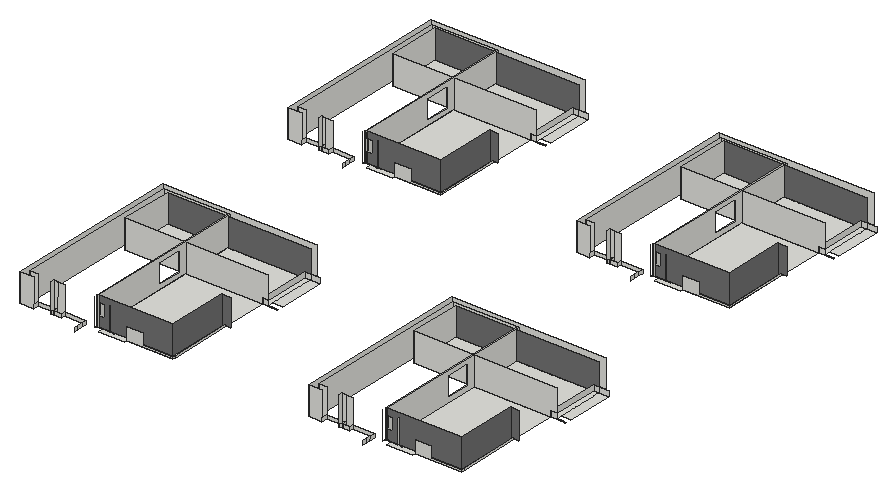
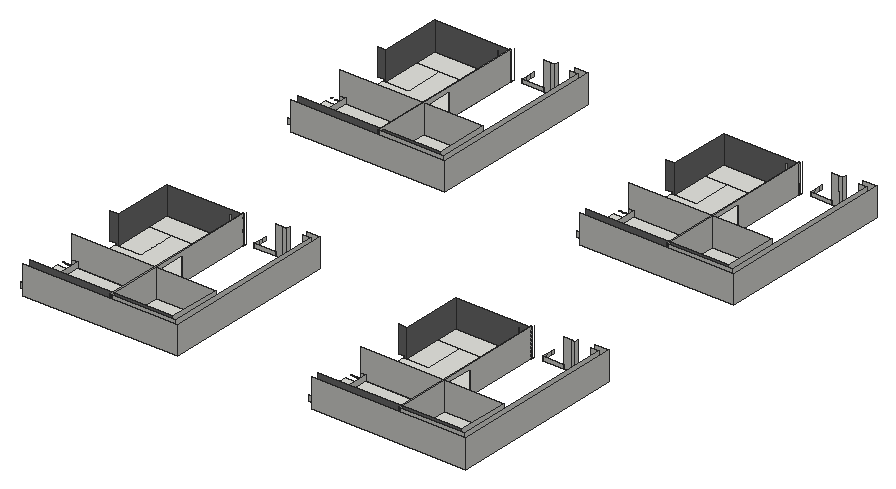
# SketchUp Ruby script. Lengths in inches.
U = 1.inch
M = Sketchup.active_model
def pt(a) = Geom::Point3d.new(a.map { |v| v * U })
def face(e, loops, mat)
  f = e.add_face(loops[0].map { |a| pt(a) })
  loops[1..].each { |l| e.add_face(l.map { |a| pt(a) }).erase! }
  f.material = f.back_material = mat if mat
  f
end
# faces: each face lists its corners as indices into pts; further lists are holes
def faces(e, pts, list, mat = nil) = list.each { |f| face(e, (f[0].is_a?(Array) ? f : [f]).map { |l| l.map { |i| pts[i] } }, mat) }
# xy, xz, yz: faces in a plane at the given z, y or x. An outline is a flat list of corners, or four numbers for a rectangle; further outlines are holes
def ring(l) = l.size == 4 ? [[l[0], l[1]], [l[2], l[1]], [l[2], l[3]], [l[0], l[3]]] : l.each_slice(2).to_a
def flat(e, list, mat, &to3) = list.each { |f| face(e, (f[0].is_a?(Array) ? f : [f]).map { |l| ring(l).map { |u, v| to3.(u, v) } }, mat) }
def xy(e, z, list, mat = nil) = flat(e, list, mat) { |x, y| [x, y, z] }
def xz(e, y, list, mat = nil) = flat(e, list, mat) { |x, z| [x, y, z] }
def yz(e, x, list, mat = nil) = flat(e, list, mat) { |y, z| [x, y, z] }
def lines(e, pts, list) = list.each { |a, b| e.add_line(pt(pts[a]), pt(pts[b])) }
# prism: a flat outline (further loops are holes) pulled along v
def prism(e, loops, v, mat = nil)
  f = face(e, loops, mat); d = Geom::Vector3d.new(v.map { |x| x * U })
  f.pushpull(f.normal.samedirection?(d) ? d.length : -d.length)
end
def box(e, o, s, mat = nil) = prism(e, [[o, [o[0] + s[0], o[1], o[2]], [o[0] + s[0], o[1] + s[1], o[2]], [o[0], o[1] + s[1], o[2]]]], [0, 0, s[2]], mat)
def at(x, y, z, deg = 0) = Geom::Transformation.translation(pt([x, y, z])) * Geom::Transformation.rotation(ORIGIN, Z_AXIS, deg.degrees)
def axes(o, x, y, z) = Geom::Transformation.new([*x, 0, *y, 0, *z, 0, *pt(o).to_a, 1])
def part(name) = M.definitions.add(name)
# library, detail: a bought-in or finely detailed component or shape, given as its bounding box
def library(name, o, s) = part(name).tap { |d| box(d.entities, o, s) }
def detail(e, o, s) = box(e.add_group.entities, o, s)
def put(e, d, t, mat = nil) = e.add_instance(d, t).tap { |i| i.material = mat if mat }
def group(e, t, mat = nil) = e.add_group.tap { |g| g.transformation = t; g.material = mat if mat }.entities
root = M.entities
M.materials.add("[Color M05]").color = [114, 114, 114]
xy(root,384,[[585.55,1810.0625,695.43,1810.0625,695.43,1822.9375,890.875,1822.9375,890.875,2095.79,878.5625,2095.79,878.5625,1837.8125,632.49,1837.8125,632.49,1834.0625,585.55,1834.0625],[1803.74,1810.0625,1913.62,1810.0625,1913.62,1822.9375,2109.0625,1822.9375,2109.0625,2095.79,2096.75,2095.79,2096.75,1837.8125,1850.67,1837.8125,1850.67,1834.0625,1803.74,1834.0625],[557.4,1832,557.88,1834.0625,557.4,1834.0625],[1775.59,1832,1776.07,1834.0625,1775.59,1834.0625],[557.88,1834.0625,557.99,1834.53,560,1834.0625,560,1837.8125,557.88,1837.8125],
  [557.88,1834.0625,557.99,1834.53,560,1834.0625],[560,1834.0625,564.5,1837.8125],[564.5,1834.0625,632.49,1835.1875],[1776.07,1834.0625,1776.18,1834.53,1778.1875,1834.0625,1778.1875,1837.8125,1776.07,1837.8125],[1776.07,1834.0625,1776.18,1834.53,1778.1875,1834.0625],
  [1778.1875,1834.0625,1782.6875,1837.8125],[1782.6875,1834.0625,1850.67,1835.1875],[564.5,1835.1875,611.65,1837.8125],[611.65,1835.1875,632.49,1837.8125],[1782.6875,1835.1875,1829.84,1837.8125],
  [1829.84,1835.1875,1850.67,1837.8125],[560,1837.8125,564.5,1838.5625],[564.5,1837.8125,611.65,1837.8125,611.65,1839.6875,632.49,1839.6875,632.49,1933.8125,564.5,1933.8125],[611.65,1837.8125,632.49,1839.6875],[632.49,1837.8125,878.5625,1933.8125],
  [1778.1875,1837.8125,1782.6875,1838.5625],[1782.6875,1837.8125,1829.84,1837.8125,1829.84,1839.6875,1850.67,1839.6875,1850.67,1933.8125,1782.6875,1933.8125],[1829.84,1837.8125,1850.67,1839.6875],[1850.67,1837.8125,2096.75,1933.8125],[560,1838.5625,564.5,2295.875],
  [1778.1875,1838.5625,1782.6875,2295.875],[564.5,1933.8125,564.5,2295.875,890.875,2295.875,890.875,2095.79,784.3125,2095.79,784.3125,1933.8125],[784.3125,1933.8125,878.5625,2095.79],[1782.6875,1933.8125,1782.6875,2295.875,2109.0625,2295.875,2109.0625,2095.79,2002.5,2095.79,2002.5,1933.8125],[2002.5,1933.8125,2096.75,2095.79],
  [308.87,2295.875,560,2518.89],[560,2295.875,564.5,2518.89],[564.5,2295.875,890.875,2518.89],[890.875,2295.875,913.875,2518.89],[1527.06,2295.875,1778.1875,2518.89],
  [1778.1875,2295.875,1782.6875,2518.89],[1782.6875,2295.875,2109.0625,2518.89],[2109.0625,2295.875,2132.0625,2518.89],[913.875,2321.98,954.6875,2518.89],[2132.0625,2321.98,2172.875,2518.89],
  [560,2518.89,564.5,2531.375],[564.5,2518.89,890.875,2531.375],[1778.1875,2518.89,1782.6875,2531.375],[1782.6875,2518.89,2109.0625,2531.375],[585.55,3224.75,695.43,3224.75,695.43,3237.625,890.875,3237.625,890.875,3510.48,878.5625,3510.48,878.5625,3252.5,632.49,3252.5,632.49,3248.75,585.55,3248.75],
  [1803.74,3224.75,1913.62,3224.75,1913.62,3237.625,2109.0625,3237.625,2109.0625,3510.48,2096.75,3510.48,2096.75,3252.5,1850.67,3252.5,1850.67,3248.75,1803.74,3248.75],[557.4,3246.6875,557.88,3248.75,557.4,3248.75],[1775.59,3246.6875,1776.07,3248.75,1775.59,3248.75],[557.88,3248.75,557.99,3249.22,560,3248.75,560,3252.5,557.88,3252.5],[557.88,3248.75,557.99,3249.22,560,3248.75],
  [560,3248.75,564.5,3252.5],[564.5,3248.75,632.49,3249.875],[1776.07,3248.75,1776.18,3249.22,1778.1875,3248.75,1778.1875,3252.5,1776.07,3252.5],[1776.07,3248.75,1776.18,3249.22,1778.1875,3248.75],[1778.1875,3248.75,1782.6875,3252.5],
  [1782.6875,3248.75,1850.67,3249.875],[564.5,3249.875,611.65,3252.5],[611.65,3249.875,632.49,3252.5],[1782.6875,3249.875,1829.84,3252.5],[1829.84,3249.875,1850.67,3252.5],
  [560,3252.5,564.5,3253.25],[564.5,3252.5,611.65,3252.5,611.65,3254.375,632.49,3254.375,632.49,3348.5,564.5,3348.5],[611.65,3252.5,632.49,3254.375],[632.49,3252.5,878.5625,3348.5],[1778.1875,3252.5,1782.6875,3253.25],
  [1782.6875,3252.5,1829.84,3252.5,1829.84,3254.375,1850.67,3254.375,1850.67,3348.5,1782.6875,3348.5],[1829.84,3252.5,1850.67,3254.375],[1850.67,3252.5,2096.75,3348.5],[560,3253.25,564.5,3710.5625],[1778.1875,3253.25,1782.6875,3710.5625],
  [564.5,3348.5,564.5,3710.5625,890.875,3710.5625,890.875,3510.48,784.3125,3510.48,784.3125,3348.5],[784.3125,3348.5,878.5625,3510.48],[1782.6875,3348.5,1782.6875,3710.5625,2109.0625,3710.5625,2109.0625,3510.48,2002.5,3510.48,2002.5,3348.5],[2002.5,3348.5,2096.75,3510.48],[308.87,3710.5625,560,3933.57],
  [560,3710.5625,564.5,3933.57],[564.5,3710.5625,890.875,3933.57],[890.875,3710.5625,913.875,3933.57],[1527.06,3710.5625,1778.1875,3933.57],[1778.1875,3710.5625,1782.6875,3933.57],
  [1782.6875,3710.5625,2109.0625,3933.57],[2109.0625,3710.5625,2132.0625,3933.57],[913.875,3736.67,954.6875,3933.57],[2132.0625,3736.67,2172.875,3933.57],[560,3933.57,564.5,3946.0625],
  [564.5,3933.57,890.875,3946.0625],[1778.1875,3933.57,1782.6875,3946.0625],[1782.6875,3933.57,2109.0625,3946.0625]])
xz(root,1799.9375,[[262.875,384,319.53,504],[1481.0625,384,1537.72,504]])
xz(root,1806.5625,[[400.54,384,400.54,399.4375,385.81,399.51,385.73,384.07],[400.54,384,400.62,399.4375,400.54,399.4375],[400.54,384,431.33,384,431.33,399.4375,400.62,399.4375],[1618.73,384,1618.73,399.4375,1604,399.51,1603.92,384.07],[1618.73,384,1618.81,399.4375,1618.73,399.4375],
  [1618.73,384,1649.52,384,1649.52,399.4375,1618.81,399.4375]])
xz(root,1822.9375,[[285.875,384,319.53,504],[319.53,384,400.54,384,385.73,384.07,385.81,399.4375,319.53,399.4375],[400.54,384,385.73,384.07,385.81,399.4375,400.54,399.4375],[400.54,384,401.14,504,386.33,504,385.81,399.4375,400.54,399.4375],[400.54,384,401.14,504,431.33,504,431.33,384],
  [431.33,384,523.04,399.4375],[695.43,384,695.43,435.5,762.28,435.5,762.28,391.25,890.875,391.25,890.875,384],[1504.0625,384,1537.72,504],[1537.72,384,1618.73,384,1603.92,384.07,1604,399.4375,1537.72,399.4375],[1618.73,384,1603.92,384.07,1604,399.4375,1618.73,399.4375],
  [1618.73,384,1619.33,504,1604.52,504,1604,399.4375,1618.73,399.4375],[1618.73,384,1619.33,504,1649.52,504,1649.52,384],[1649.52,384,1741.23,399.4375],[1913.62,384,1913.62,435.5,1980.47,435.5,1980.47,391.25,2109.0625,391.25,2109.0625,384]])
xz(root,1834.0625,[[560,384,564.5,504],[1778.1875,384,1782.6875,504]])
xz(root,1837.8125,[[557.88,384,560,424.93],[560,384,564.5,424.93],[1776.07,384,1778.1875,424.93],[1778.1875,384,1782.6875,424.93]])
xz(root,1837.8125,[[564.5,384,878.5625,384,878.5625,504,564.5,504,564.5,477.21,589.71,477.21,589.71,424.93,564.5,424.93],[1782.6875,384,2096.75,384,2096.75,504,1782.6875,504,1782.6875,477.21,1807.9,477.21,1807.9,424.93,1782.6875,424.93]],"[Color M05]")
xz(root,1838.5625,[[560,384,564.5,504],[1778.1875,384,1782.6875,504]])
xz(root,2095.79,[[878.5625,384,890.875,384,890.875,391.25,913.875,391.25,913.875,504,878.5625,504],[2096.75,384,2109.0625,384,2109.0625,391.25,2132.0625,391.25,2132.0625,504,2096.75,504]],"[Color M05]")
xz(root,2295.875,[[308.87,384,308.87,504,913.875,504,913.875,408.0625,890.875,408.0625,890.875,384],[890.875,384,913.875,408.0625],[913.875,384,930.75,385.75],[930.75,384,954.6875,385.75],[1527.06,384,1527.06,504,2132.0625,504,2132.0625,408.0625,2109.0625,408.0625,2109.0625,384],
  [2109.0625,384,2132.0625,408.0625],[2132.0625,384,2148.9375,385.75],[2148.9375,384,2172.875,385.75]])
xz(root,2518.89,[[890.875,384,913.875,408.0625],[913.875,384,954.6875,408.0625],[2109.0625,384,2132.0625,408.0625],[2132.0625,384,2172.875,408.0625]])
xz(root,2518.89,[[308.87,384,890.875,384,890.875,408.0625,913.875,408.0625,913.875,504,308.87,504],[1527.06,384,2109.0625,384,2109.0625,408.0625,2132.0625,408.0625,2132.0625,504,1527.06,504]],"[Color M05]")
xz(root,2531.375,[[285.875,384,560,504],[560,384,564.5,504],[1504.0625,384,1778.1875,504],[1778.1875,384,1782.6875,504]])
xz(root,2554.375,[[262.875,384,913.875,504],[1481.0625,384,2132.0625,504]])
xz(root,3214.625,[[262.875,384,319.53,504],[1481.0625,384,1537.72,504]])
xz(root,3221.25,[[400.54,384,400.54,399.4375,385.81,399.51,385.73,384.07],[400.54,384,400.62,399.4375,400.54,399.4375],[400.54,384,431.33,384,431.33,399.4375,400.62,399.4375],[1618.73,384,1618.73,399.4375,1604,399.51,1603.92,384.07],[1618.73,384,1618.81,399.4375,1618.73,399.4375],
  [1618.73,384,1649.52,384,1649.52,399.4375,1618.81,399.4375]])
xz(root,3237.625,[[285.875,384,319.53,504],[319.53,384,400.54,384,385.73,384.07,385.81,399.4375,319.53,399.4375],[400.54,384,385.73,384.07,385.81,399.4375,400.54,399.4375],[400.54,384,401.14,504,386.33,504,385.81,399.4375,400.54,399.4375],[400.54,384,401.14,504,431.33,504,431.33,384],
  [431.33,384,523.04,399.4375],[695.43,384,695.43,435.5,762.28,435.5,762.28,391.25,890.875,391.25,890.875,384],[1504.0625,384,1537.72,504],[1537.72,384,1618.73,384,1603.92,384.07,1604,399.4375,1537.72,399.4375],[1618.73,384,1603.92,384.07,1604,399.4375,1618.73,399.4375],
  [1618.73,384,1619.33,504,1604.52,504,1604,399.4375,1618.73,399.4375],[1618.73,384,1619.33,504,1649.52,504,1649.52,384],[1649.52,384,1741.23,399.4375],[1913.62,384,1913.62,435.5,1980.47,435.5,1980.47,391.25,2109.0625,391.25,2109.0625,384]])
xz(root,3248.75,[[560,384,564.5,504],[1778.1875,384,1782.6875,504]])
xz(root,3252.5,[[557.88,384,560,424.93],[560,384,564.5,424.93],[1776.07,384,1778.1875,424.93],[1778.1875,384,1782.6875,424.93]])
xz(root,3252.5,[[564.5,384,878.5625,384,878.5625,504,564.5,504,564.5,477.21,589.71,477.21,589.71,424.93,564.5,424.93],[1782.6875,384,2096.75,384,2096.75,504,1782.6875,504,1782.6875,477.21,1807.9,477.21,1807.9,424.93,1782.6875,424.93]],"[Color M05]")
xz(root,3253.25,[[560,384,564.5,504],[1778.1875,384,1782.6875,504]])
xz(root,3510.48,[[878.5625,384,890.875,384,890.875,391.25,913.875,391.25,913.875,504,878.5625,504],[2096.75,384,2109.0625,384,2109.0625,391.25,2132.0625,391.25,2132.0625,504,2096.75,504]],"[Color M05]")
xz(root,3710.5625,[[308.87,384,308.87,504,913.875,504,913.875,408.0625,890.875,408.0625,890.875,384],[890.875,384,913.875,408.0625],[913.875,384,930.75,385.75],[930.75,384,954.6875,385.75],[1527.06,384,1527.06,504,2132.0625,504,2132.0625,408.0625,2109.0625,408.0625,2109.0625,384],
  [2109.0625,384,2132.0625,408.0625],[2132.0625,384,2148.9375,385.75],[2148.9375,384,2172.875,385.75]])
xz(root,3933.57,[[890.875,384,913.875,408.0625],[913.875,384,954.6875,408.0625],[2109.0625,384,2132.0625,408.0625],[2132.0625,384,2172.875,408.0625]])
xz(root,3933.57,[[308.87,384,890.875,384,890.875,408.0625,913.875,408.0625,913.875,504,308.87,504],[1527.06,384,2109.0625,384,2109.0625,408.0625,2132.0625,408.0625,2132.0625,504,1527.06,504]],"[Color M05]")
xz(root,3946.0625,[[285.875,384,560,504],[560,384,564.5,504],[1504.0625,384,1778.1875,504],[1778.1875,384,1782.6875,504]])
xz(root,3969.0625,[[262.875,384,913.875,504],[1481.0625,384,2132.0625,504]])
yz(root,262.875,[[1799.9375,384,2554.375,504],[3214.625,384,3969.0625,504]])
yz(root,285.875,[[1822.9375,384,2531.375,504],[3237.625,384,3946.0625,504]])
yz(root,308.87,[[2295.875,384,2518.89,504],[3710.5625,384,3933.57,504]])
yz(root,319.53,[[1799.9375,384,1822.9375,399.4375],[3214.625,384,3237.625,399.4375]])
yz(root,400.54,[[1806.5625,384,1822.9375,399.4375],[3221.25,384,3237.625,399.4375]])
yz(root,431.33,[[1806.5625,384,1822.9375,399.4375],[3221.25,384,3237.625,399.4375]])
yz(root,523.04,[[1763.25,384,1799.9375,399.4375],[1799.9375,384,1822.9375,399.4375],[3177.9375,384,3214.625,399.4375],[3214.625,384,3237.625,399.4375]])
yz(root,560,[[1834.0625,384,1837.8125,504],[1837.8125,384,1838.5625,504],[[1838.5625,384,2531.375,504],[2156.01,401.36,2266.33,487.04]],[3248.75,384,3252.5,504],[3252.5,384,3253.25,504],
  [[3253.25,384,3946.0625,504],[3570.7,401.36,3681.01,487.04]]])
yz(root,564.5,[[1834.0625,384,1837.8125,504],[1837.8125,384,1838.5625,424.93],[[1838.5625,384,2531.375,384,2531.375,504,1838.5625,504,1838.5625,477.21,1847.4375,477.21,1847.4375,424.93,1838.5625,424.93],[2156.01,401.36,2266.33,487.04]],[3248.75,384,3252.5,504],[3252.5,384,3253.25,424.93],
  [[3253.25,384,3946.0625,384,3946.0625,504,3253.25,504,3253.25,477.21,3262.125,477.21,3262.125,424.93,3253.25,424.93],[3570.7,401.36,3681.01,487.04]]])
yz(root,611.65,[[1835.1875,384,1839.6875,481.8125],[3249.875,384,3254.375,481.8125]])
yz(root,878.5625,[[1837.8125,384,2095.79,504],[3252.5,384,3510.48,504]],"[Color M05]")
yz(root,890.875,[[1822.9375,384,1835.1875,391.25],[1835.1875,384,2095.79,391.25],[2295.875,384,2518.89,408.0625],[3237.625,384,3249.875,391.25],[3249.875,384,3510.48,391.25],
  [3710.5625,384,3933.57,408.0625]])
yz(root,1481.0625,[[1799.9375,384,2554.375,504],[3214.625,384,3969.0625,504]])
yz(root,1504.0625,[[1822.9375,384,2531.375,504],[3237.625,384,3946.0625,504]])
yz(root,1527.06,[[2295.875,384,2518.89,504],[3710.5625,384,3933.57,504]])
yz(root,1537.72,[[1799.9375,384,1822.9375,399.4375],[3214.625,384,3237.625,399.4375]])
yz(root,1618.73,[[1806.5625,384,1822.9375,399.4375],[3221.25,384,3237.625,399.4375]])
yz(root,1649.52,[[1806.5625,384,1822.9375,399.4375],[3221.25,384,3237.625,399.4375]])
yz(root,1741.23,[[1763.25,384,1799.9375,399.4375],[1799.9375,384,1822.9375,399.4375],[3177.9375,384,3214.625,399.4375],[3214.625,384,3237.625,399.4375]])
yz(root,1778.1875,[[1834.0625,384,1837.8125,504],[1837.8125,384,1838.5625,504],[[1838.5625,384,2531.375,504],[2156.01,401.36,2266.33,487.04]],[3248.75,384,3252.5,504],[3252.5,384,3253.25,504],
  [[3253.25,384,3946.0625,504],[3570.7,401.36,3681.01,487.04]]])
yz(root,1782.6875,[[1834.0625,384,1837.8125,504],[1837.8125,384,1838.5625,424.93],[[1838.5625,384,2531.375,384,2531.375,504,1838.5625,504,1838.5625,477.21,1847.4375,477.21,1847.4375,424.93,1838.5625,424.93],[2156.01,401.36,2266.33,487.04]],[3248.75,384,3252.5,504],[3252.5,384,3253.25,424.93],
  [[3253.25,384,3946.0625,384,3946.0625,504,3253.25,504,3253.25,477.21,3262.125,477.21,3262.125,424.93,3253.25,424.93],[3570.7,401.36,3681.01,487.04]]])
yz(root,1829.84,[[1835.1875,384,1839.6875,481.8125],[3249.875,384,3254.375,481.8125]])
yz(root,2096.75,[[1837.8125,384,2095.79,504],[3252.5,384,3510.48,504]],"[Color M05]")
yz(root,2109.0625,[[1822.9375,384,1835.1875,391.25],[1835.1875,384,2095.79,391.25],[2295.875,384,2518.89,408.0625],[3237.625,384,3249.875,391.25],[3249.875,384,3510.48,391.25],
  [3710.5625,384,3933.57,408.0625]])
p = [[400.54,1822.9375,384],[400.54,1806.5625,384],[385.73,1806.5625,384.07],[385.73,1822.9375,384.07],[1618.73,1822.9375,384],[1618.73,1806.5625,384],
  [1603.92,1806.5625,384.07],[1603.92,1822.9375,384.07],[400.54,3237.625,384],[400.54,3221.25,384],[385.73,3221.25,384.07],[385.73,3237.625,384.07],
  [1618.73,3237.625,384],[1618.73,3221.25,384],[1603.92,3221.25,384.07],[1603.92,3237.625,384.07],[385.81,1806.5625,399.51],[386.33,1806.5625,504.07],
  [386.33,1822.9375,504.07],[386.33,1822.9375,504],[385.81,1822.9375,399.4375],[1604,1806.5625,399.51],[1604.52,1806.5625,504.07],[1604.52,1822.9375,504.07],
  [1604.52,1822.9375,504],[1604,1822.9375,399.4375],[385.81,3221.25,399.51],[386.33,3221.25,504.07],[386.33,3237.625,504.07],[386.33,3237.625,504],
  [385.81,3237.625,399.4375],[1604,3221.25,399.51],[1604.52,3221.25,504.07],[1604.52,3237.625,504.07],[1604.52,3237.625,504],[1604,3237.625,399.4375],
  [1775.59,1822.9375,384],[1778.1875,1834.0625,384],[1773.58,1823.41,384],[1775.59,1832,384],[1773.58,1823.41,504],[1741.23,1778.3125,384],
  [1741.23,1778.3125,399.4375],[557.4,1822.9375,384],[560,1834.0625,384],[555.39,1823.41,384],[557.4,1832,384],[555.39,1823.41,504],
  [523.04,1778.3125,384],[523.04,1778.3125,399.4375],[1741.23,3193,384],[1741.23,3193,399.4375],[1775.59,3237.625,384],[1778.1875,3248.75,384],
  [1773.58,3238.09,504],[1773.58,3238.09,384],[1775.59,3246.6875,384],[557.4,3237.625,384],[560,3248.75,384],[555.39,3238.09,384],
  [557.4,3246.6875,384],[555.39,3238.09,504],[523.04,3193,384],[523.04,3193,399.4375]]
faces(root,p,[[0,1,2,3],[4,5,6,7],[8,9,10,11],[12,13,14,15],[3,2,16,17,18,19,20],[7,6,21,22,23,24,25],[11,10,26,27,28,29,30],[15,14,31,32,33,34,35]])
lines(root,p,[[36,37],[38,39],[40,38],[41,42],[43,44],[45,46],[47,45],[48,49],[50,51],[52,53],[54,55],[55,56],
  [57,58],[59,60],[61,59],[62,63]])
